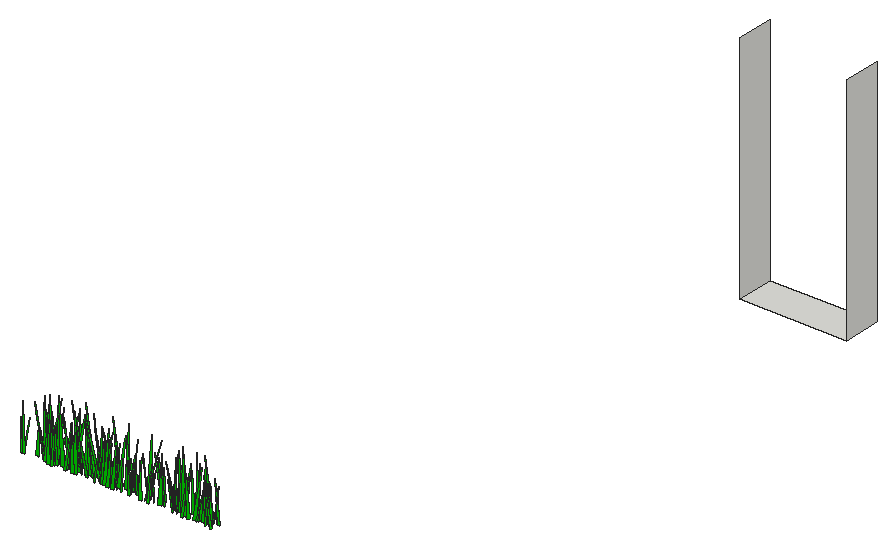
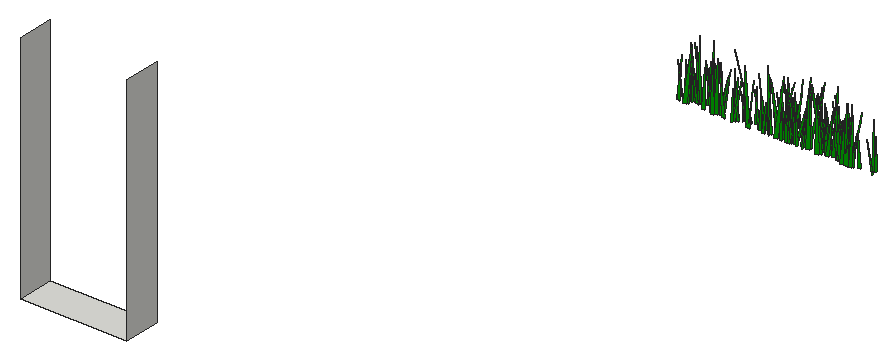
# SketchUp Ruby script. Lengths in inches.
U = 1.inch
M = Sketchup.active_model
def pt(a) = Geom::Point3d.new(a.map { |v| v * U })
def face(e, loops, mat)
  f = e.add_face(loops[0].map { |a| pt(a) })
  loops[1..].each { |l| e.add_face(l.map { |a| pt(a) }).erase! }
  f.material = f.back_material = mat if mat
  f
end
# faces: each face lists its corners as indices into pts; further lists are holes
def faces(e, pts, list, mat = nil) = list.each { |f| face(e, (f[0].is_a?(Array) ? f : [f]).map { |l| l.map { |i| pts[i] } }, mat) }
# xy, xz, yz: faces in a plane at the given z, y or x. An outline is a flat list of corners, or four numbers for a rectangle; further outlines are holes
def ring(l) = l.size == 4 ? [[l[0], l[1]], [l[2], l[1]], [l[2], l[3]], [l[0], l[3]]] : l.each_slice(2).to_a
def flat(e, list, mat, &to3) = list.each { |f| face(e, (f[0].is_a?(Array) ? f : [f]).map { |l| ring(l).map { |u, v| to3.(u, v) } }, mat) }
def xy(e, z, list, mat = nil) = flat(e, list, mat) { |x, y| [x, y, z] }
def xz(e, y, list, mat = nil) = flat(e, list, mat) { |x, z| [x, y, z] }
def yz(e, x, list, mat = nil) = flat(e, list, mat) { |y, z| [x, y, z] }
def lines(e, pts, list) = list.each { |a, b| e.add_line(pt(pts[a]), pt(pts[b])) }
# prism: a flat outline (further loops are holes) pulled along v
def prism(e, loops, v, mat = nil)
  f = face(e, loops, mat); d = Geom::Vector3d.new(v.map { |x| x * U })
  f.pushpull(f.normal.samedirection?(d) ? d.length : -d.length)
end
def box(e, o, s, mat = nil) = prism(e, [[o, [o[0] + s[0], o[1], o[2]], [o[0] + s[0], o[1] + s[1], o[2]], [o[0], o[1] + s[1], o[2]]]], [0, 0, s[2]], mat)
def at(x, y, z, deg = 0) = Geom::Transformation.translation(pt([x, y, z])) * Geom::Transformation.rotation(ORIGIN, Z_AXIS, deg.degrees)
def axes(o, x, y, z) = Geom::Transformation.new([*x, 0, *y, 0, *z, 0, *pt(o).to_a, 1])
def part(name) = M.definitions.add(name)
# library, detail: a bought-in or finely detailed component or shape, given as its bounding box
def library(name, o, s) = part(name).tap { |d| box(d.entities, o, s) }
def detail(e, o, s) = box(e.add_group.entities, o, s)
def put(e, d, t, mat = nil) = e.add_instance(d, t).tap { |i| i.material = mat if mat }
def group(e, t, mat = nil) = e.add_group.tap { |g| g.transformation = t; g.material = mat if mat }.entities
root = M.entities
M.materials.add("[Color G06]").color = [0, 204, 0]
c1 = part("fur_instance\#9")
p = [[0.8125,0,1.79],[0.67,-0.02,1.48],[0,-0.11,0],[0,0.11,0]]
faces(c1.entities,p,[[0,1,2,3]])
xy(root,4.64,[[144.35,175.125,174.23,185.625]])
yz(root,144.35,[[175.125,4.64,185.625,70.2]])
yz(root,174.23,[[175.125,4.64,185.625,70.2]])
put(root,c1,axes([117.61,23,4.28],[-2.5599,0.32054,0.39993],[2.31118,0.35695,0.17964],[0.11843,-0.03742,5.13894]),"[Color G06]")
put(root,c1,axes([72.84,23.15,4.28],[2.39176,-0.2676,1.34014],[-1.98531,-0.34895,-0.08977],[-0.73841,0.07143,4.58218]),"[Color G06]")
put(root,c1,axes([84.67,23.125,4.28],[2.95899,0.07959,1.00137],[0.60026,-0.42215,-0.10781],[-0.64369,-0.02781,4.50266]),"[Color G06]")
put(root,c1,axes([99.72,23.21,4.28],[2.01452,-0.26444,1.03727],[-1.95316,-0.28988,-0.01622],[-0.51301,0.0652,4.135]),"[Color G06]")
put(root,c1,axes([115.85,23.19,4.28],[-2.65021,0.2148,1.87506],[1.74432,0.39119,0.35918],[0.95084,-0.11895,4.56729]),"[Color G06]")
put(root,c1,axes([88.24,23.3125,4.28],[2.48366,-0.43512,0.95898],[-3.15902,-0.35104,-0.02176],[-0.41112,0.06872,5.96054]),"[Color G06]")
put(root,c1,axes([76.27,23.26,4.28],[2.97995,-0.33517,0.86688],[-2.45565,-0.41597,0.38077],[-0.28869,0.07863,5.70926]),"[Color G06]")
put(root,c1,axes([109.36,23.07,4.28],[0.6028,0.39995,0.34159],[2.87417,-0.0822,-0.27409],[0.1331,-0.0364,4.37174]),"[Color G06]")
put(root,c1,axes([71.66,23.17,4.28],[-1.43471,0.42994,1.50699],[3.19984,0.21282,-0.17016],[0.53282,-0.12042,5.07971]),"[Color G06]")
put(root,c1,axes([89.84,23.08,4.28],[1.51874,0.50728,0.66766],[3.65066,-0.21537,0.24767],[-0.32585,-0.04847,5.88662]),"[Color G06]")
put(root,c1,axes([110.98,23.25,4.28],[-2.84036,0.2913,2.00087],[2.29731,0.41596,0.32806],[0.93728,-0.13677,5.25939]),"[Color G06]")
put(root,c1,axes([87.25,23.33,4.28],[-2.79469,0.4392,4.2365],[3.72814,0.47991,-0.22183],[2.01398,-0.27892,6.2894]),"[Color G06]")
put(root,c1,axes([78.32,23.36,4.28],[0.29829,-0.52756,2.06636],[-4.02276,-0.04888,-0.13656],[-0.20558,0.19108,5.67031]),"[Color G06]")
put(root,c1,axes([89.44,23.41,4.28],[-2.8058,-0.48055,1.79717],[-3.58951,0.40162,-0.1816],[0.66131,0.14106,6.6393]),"[Color G06]")
put(root,c1,axes([94.18,23.34,4.28],[-2.1101,-0.2329,1.69497],[-1.84814,0.3149,-0.16881],[0.81239,0.11146,4.01849]),"[Color G06]")
put(root,c1,axes([106.39,23.42,4.28],[-2.33762,-0.19114,0.64303],[-1.40579,0.32795,-0.21743],[0.2961,0.04802,4.04423]),"[Color G06]")
put(root,c1,axes([97.49,23.3125,4.28],[-0.5252,0.45283,1.11862],[3.33154,0.07389,0.05775],[0.08037,-0.1039,4.91617]),"[Color G06]")
put(root,c1,axes([112.3,23.65,4.28],[3.10487,-0.60042,0.08751],[-4.30615,-0.43296,0.02328],[-0.02161,0.00789,7.93391]),"[Color G06]")
put(root,c1,axes([79.09,23.48,4.28],[2.73116,-0.57067,2.98564],[-4.37171,-0.41953,-0.2786],[-1.27545,0.21596,7.34815]),"[Color G06]")
put(root,c1,axes([73.05,23.31,4.28],[-1.69569,0.40002,0.32371],[2.8636,0.23806,-0.28629],[0.27528,-0.01234,4.97218]),"[Color G06]")
put(root,c1,axes([88.36,23.54,4.28],[2.56578,0.37607,3.21461],[3.01226,-0.42641,0.35992],[-1.68094,-0.19011,5.55175]),"[Color G06]")
put(root,c1,axes([91.88,23.63,4.28],[2.03788,-0.29646,0.84145],[-2.12734,-0.29287,-0.34437],[-0.55775,0.03387,4.38793]),"[Color G06]")
put(root,c1,axes([63.83,23.51,4.28],[2.2039,-0.21291,2.10143],[-1.78737,-0.34006,0.22942],[-1.05518,0.13134,4.00054]),"[Color G06]")
put(root,c1,axes([86.43,23.5,4.28],[-2.44167,-0.2565,2.83012],[-2.24312,0.39123,-0.24954],[1.39201,0.18052,4.56211]),"[Color G06]")
put(root,c1,axes([82.1,23.6875,4.28],[-4.64314,-0.43907,0.64752],[-3.16885,0.64777,-0.29859],[0.24588,0.05701,8.37937]),"[Color G06]")
put(root,c1,axes([107.46,23.6,4.28],[-3.35251,-0.15897,0.34434],[-1.15268,0.4672,-0.29086],[0.15501,0.03608,5.28434]),"[Color G06]")
put(root,c1,axes([109.38,23.45,4.28],[-2.29398,0.72773,2.34567],[5.38397,0.33938,-0.33396],[0.84324,-0.18719,8.51349]),"[Color G06]")
put(root,c1,axes([78.55,23.77,4.28],[4.51424,-0.47738,0.28232],[-3.42474,-0.6299,-0.03153],[-0.16326,0.01357,8.46749]),"[Color G06]")
put(root,c1,axes([90.55,23.625,4.28],[-5.29936,0.01222,0.2267],[0.08741,0.73927,-0.01237],[0.1518,0.0008,7.92136]),"[Color G06]")
put(root,c1,axes([98.36,23.65,4.28],[6.18917,0.0656,0.13916],[0.47387,-0.86239,-0.37808],[-0.07359,-0.03616,9.26914]),"[Color G06]")
put(root,c1,axes([113.07,23.53,4.28],[2.59838,0.28438,0.02851],[2.03238,-0.36141,0.37525],[-0.16998,0.0259,4.92249]),"[Color G06]")
put(root,c1,axes([115.7,23.68,4.28],[2.75461,0.17443,2.20644],[1.41082,-0.42616,-0.06434],[-1.32427,-0.09119,4.5211]),"[Color G06]")
put(root,c1,axes([64.5,23.63,4.28],[-2.96816,0.41781,2.14015],[3.10848,0.44379,-0.32288],[1.16852,-0.11928,6.29513]),"[Color G06]")
put(root,c1,axes([87.4375,23.69,4.28],[-2.98027,0.20442,1.90008],[1.56465,0.44533,-0.02175],[1.14765,-0.0763,4.96387]),"[Color G06]")
put(root,c1,axes([70.33,23.72,4.28],[-4.0538,0.18348,3.82784],[1.40302,0.66444,-0.33958],[2.51442,-0.07494,6.36079]),"[Color G06]")
put(root,c1,axes([116.875,23.62,4.28],[-0.12835,0.48306,0.56522],[3.48458,0.01828,-0.02747],[0.03248,-0.0526,5.18091]),"[Color G06]")
put(root,c1,axes([86.54,23.82,4.28],[4.87915,-0.01885,0.99327],[-0.12733,-0.68662,-0.09972],[-0.66613,-0.00682,7.29437]),"[Color G06]")
put(root,c1,axes([113,23.84,4.28],[3.5428,0.53992,3.61843],[4.24445,-0.54697,0.09275],[-1.68464,-0.24262,7.84323]),"[Color G06]")
put(root,c1,axes([85.75,23.88,4.28],[3.4918,0.04867,1.61056],[0.43542,-0.50724,-0.34774],[-1.04569,-0.04869,5.23322]),"[Color G06]")
put(root,c1,axes([73.4375,23.89,4.28],[-2.37338,0.25729,1.7778],[2.01847,0.35181,0.17021],[0.86325,-0.11522,4.48981]),"[Color G06]")
put(root,c1,axes([93.93,23.86,4.28],[2.75429,-0.38398,3.83172],[-3.35008,-0.45195,0.17627],[-1.7124,0.26657,5.81822]),"[Color G06]")
put(root,c1,axes([80.56,23.96,4.28],[-6.04895,-0.02529,1.8238],[-0.20795,0.86023,-0.17053],[1.21603,0.02132,9.04305]),"[Color G06]")
put(root,c1,axes([69.71,24.09,4.28],[-1.78004,-0.30337,0.47503],[-2.17273,0.25145,0.26042],[0.3366,0.01875,4.19313]),"[Color G06]")
put(root,c1,axes([89.21,24.04,4.28],[2.18577,-0.21646,0.93995],[-1.58102,-0.31425,-0.10069],[-0.55267,0.0429,4.00551]),"[Color G06]")
put(root,c1,axes([74.93,24.22,4.28],[-1.3467,-0.84024,1.52468],[-6.10648,0.19083,0.03274],[0.24417,0.13815,9.22785]),"[Color G06]")
put(root,c1,axes([88.76,24.09,4.28],[-2.07942,-0.3279,1.15131],[-2.37477,0.30387,0.36085],[0.69502,0.05726,4.67753]),"[Color G06]")
put(root,c1,axes([69.97,24.05,4.28],[-4.84878,-0.02816,0.938],[-0.17519,0.68124,0.32664],[0.6356,-0.02706,7.24578]),"[Color G06]")
put(root,c1,axes([98.89,24.06,4.28],[-3.72793,-0.04329,1.4862],[-0.30147,0.53802,0.11098],[0.99715,0.00083,5.58985]),"[Color G06]")
put(root,c1,axes([76.14,23.92,4.28],[1.36909,0.58691,0.09506],[4.20916,-0.19079,-0.09339],[0.03975,-0.01113,6.61423]),"[Color G06]")
put(root,c1,axes([106.54,24.34,4.28],[-3.38436,-0.37645,0.00598],[-2.69604,0.47135,0.32596],[0.13913,-0.02343,6.46208]),"[Color G06]")
put(root,c1,axes([114.72,23.98,4.28],[1.17303,0.70372,1.07038],[5.08413,-0.16884,0.30605],[-0.36337,-0.09067,7.73744]),"[Color G06]")
put(root,c1,axes([106.84,24.3125,4.28],[-1.53866,-0.44725,0.95187],[-3.2292,0.22327,0.39138],[0.51459,0.06381,5.30223]),"[Color G06]")
put(root,c1,axes([88.91,24.2,4.28],[1.79576,0.2418,1.9153],[1.90952,-0.28635,0.15374],[-1.0014,-0.11243,3.72775]),"[Color G06]")
put(root,c1,axes([114.63,24.17,4.28],[-3.18706,0.1035,2.27879],[0.71296,0.49247,-0.34214],[1.53862,-0.01381,4.87879]),"[Color G06]")
put(root,c1,axes([115.71,24.375,4.28],[-0.3016,-0.4986,0.55212],[-3.5893,0.04458,0.2449],[0.19516,0.04935,5.35734]),"[Color G06]")
put(root,c1,axes([100.37,24.26,4.28],[-2.96972,-0.03428,1.75489],[-0.24888,0.44524,0.05842],[1.17354,0.00767,4.45326]),"[Color G06]")
put(root,c1,axes([113,24.23,4.28],[-4.05303,-0.20678,3.44647],[-1.75316,0.63671,-0.21697],[2.10782,0.13198,6.44659]),"[Color G06]")
put(root,c1,axes([85.75,24.32,4.28],[-5.18997,-0.27488,1.84227],[-2.02957,0.74076,-0.07525],[1.13396,0.06775,8.29709]),"[Color G06]")
put(root,c1,axes([73.56,24.25,4.28],[2.69049,0.15872,0.20713],[1.14622,-0.37362,-0.36884],[-0.03091,-0.03923,4.35057]),"[Color G06]")
put(root,c1,axes([88.79,24.27,4.28],[2.55794,0.15734,0.56626],[1.14414,-0.35956,-0.06774],[-0.32814,-0.02716,4.17792]),"[Color G06]")
put(root,c1,axes([107.73,24.39,4.28],[-1.14535,0.46018,3.07666],[3.79808,0.19682,-0.22355],[0.83835,-0.263,5.21605]),"[Color G06]")
put(root,c1,axes([103.24,24.4,4.28],[-2.75886,-0.25135,1.55607],[-1.87261,0.40495,0.09779],[0.90897,0.07138,4.92436]),"[Color G06]")
put(root,c1,axes([81.54,24.3,4.28],[0.50592,0.61722,2.12596],[4.63739,-0.08122,0.24376],[-0.33152,-0.19423,6.65401]),"[Color G06]")
put(root,c1,axes([113.46,24.27,4.28],[0.96738,0.38767,0.31174],[2.78709,-0.13373,-0.21498],[0.06773,-0.03405,4.39416]),"[Color G06]")
put(root,c1,axes([85.29,24.35,4.28],[-5.38822,0.22331,0.07516],[1.6022,0.75082,0.30536],[-0.01004,-0.02931,8.39569]),"[Color G06]")
put(root,c1,axes([102.27,24.19,4.28],[0.65066,0.65996,0.03595],[4.72906,-0.09079,0.27878],[-0.18807,0.00022,7.13452]),"[Color G06]")
put(root,c1,axes([67.5,24.6,4.28],[0.22864,-0.39622,0.60995],[-2.8647,-0.02784,0.32113],[0.18371,0.05899,4.24833]),"[Color G06]")
put(root,c1,axes([90.35,24.34,4.28],[2.83915,0.54653,0.84565],[3.95512,-0.39615,-0.25015],[-0.19527,-0.07764,7.22881]),"[Color G06]")
put(root,c1,axes([77.11,24.45,4.28],[2.98341,-0.21861,2.81273],[-1.91767,-0.46576,0.38502],[-1.52383,0.15814,5.02233]),"[Color G06]")
put(root,c1,axes([85.95,24.67,4.28],[-3.18494,-0.45944,0.4711],[-3.29927,0.44556,0.09351],[0.26415,0.02552,6.84827]),"[Color G06]")
put(root,c1,axes([107.7,24.47,4.28],[3.31788,0.20952,0.06508],[1.5022,-0.4627,0.04798],[-0.05291,0.00157,5.44337]),"[Color G06]")
put(root,c1,axes([76.42,24.51,4.28],[4.9796,0.17635,1.10664],[1.27508,-0.70164,0.0279],[-0.7223,-0.02287,7.67858]),"[Color G06]")
put(root,c1,axes([70.89,24.46,4.28],[0.57605,0.4763,0.65461],[3.43102,-0.08469,0.33416],[-0.29491,-0.05487,5.16632]),"[Color G06]")
put(root,c1,axes([79.05,24.65,4.28],[-1.49114,-0.34433,1.32385],[-2.59194,0.21529,-0.08889],[0.40453,0.1102,4.31027]),"[Color G06]")
put(root,c1,axes([116,24.65,4.28],[-3.5417,-0.23177,1.27947],[-1.73909,0.50227,-0.30124],[0.6863,0.07669,5.83947]),"[Color G06]")
put(root,c1,axes([83.03,24.58,4.28],[-2.47971,0.20071,0.92667],[1.46025,0.35466,-0.09582],[0.56903,-0.03548,4.28413]),"[Color G06]")
put(root,c1,axes([90.32,24.67,4.28],[-2.60091,-0.24776,1.90599],[-1.94655,0.38821,-0.13627],[0.99709,0.11159,4.70573]),"[Color G06]")
put(root,c1,axes([94.09,24.65,4.28],[4.61964,0.04994,1.88172],[0.32091,-0.66756,0.27547],[-1.26904,0.01299,6.91963]),"[Color G06]")
put(root,c1,axes([95.65,24.66,4.28],[2.41199,0.30614,1.1997],[2.26998,-0.34515,-0.07665],[-0.558,-0.08078,4.87398]),"[Color G06]")
put(root,c1,axes([83.55,24.76,4.28],[-5.98442,0.19047,2.0085],[1.44632,0.8521,0.34354],[1.25689,-0.07366,9.16773]),"[Color G06]")
put(root,c1,axes([99.21,24.78,4.28],[2.7154,0.04043,0.60274],[0.29582,-0.38271,-0.02778],[-0.399,-0.00858,4.08134]),"[Color G06]")
put(root,c1,axes([79.73,24.8,4.28],[-3.0244,0.07305,0.11029],[0.52822,0.42023,0.384],[0.0286,-0.03706,4.57139]),"[Color G06]")
put(root,c1,axes([106.09,24.83,4.28],[2.41017,-0.46009,2.45395],[-3.53744,-0.36554,-0.11224],[-1.0337,0.17819,6.10574]),"[Color G06]")
put(root,c1,axes([95.31,24.81,4.28],[1.61229,-0.25452,1.94053],[-2.01281,-0.26251,-0.21964],[-0.98282,0.12007,3.63321]),"[Color G06]")
put(root,c1,axes([88.8,24.7,4.28],[2.21731,0.4462,0.75612],[3.23855,-0.30745,-0.372],[-0.08125,-0.0778,5.80645]),"[Color G06]")
put(root,c1,axes([92.3,24.89,4.28],[2.86346,-0.65702,2.69477],[-4.96502,-0.41825,0.07073],[-0.89383,0.21846,8.24005]),"[Color G06]")
put(root,c1,axes([85.125,24.93,4.28],[-0.01838,-0.5965,1.69919],[-4.42104,0.01009,0.29999],[0.21256,0.15824,6.38626]),"[Color G06]")
put(root,c1,axes([69.36,25,4.28],[1.35839,-0.39591,0.00678],[-2.83913,-0.18941,0.03446],[0.01884,0.00196,4.70392]),"[Color G06]")
put(root,c1,axes([108.24,24.9,4.28],[4.04824,-0.11308,1.15367],[-0.85326,-0.57307,0.2353],[-0.72486,0.04303,6.1661]),"[Color G06]")
put(root,c1,axes([76.33,24.75,4.28],[-2.71708,0.45907,0.5274],[3.29649,0.38103,-0.16376],[0.30934,-0.02818,6.37756]),"[Color G06]")
put(root,c1,axes([101.33,24.875,4.28],[1.9813,0.31172,1.12863],[2.31245,-0.28386,-0.06167],[-0.46899,-0.08273,4.46399]),"[Color G06]")
put(root,c1,axes([116.125,24.9375,4.28],[-2.10143,-0.26608,1.42529],[-2.06902,0.29967,-0.38757],[0.51916,0.11726,4.22457]),"[Color G06]")
put(root,c1,axes([81.7,24.89,4.28],[-2.08585,0.61709,2.60961],[4.70231,0.30776,0.0356],[0.72156,-0.22174,7.31179]),"[Color G06]")
put(root,c1,axes([73.58,24.9375,4.28],[-3.46109,-0.34535,3.67224],[-2.75104,0.56698,0.33347],[2.14535,0.16989,6.35203]),"[Color G06]")
put(root,c1,axes([116.71,25.03,4.28],[3.29551,0.01778,1.16478],[0.1769,-0.47112,-0.29199],[-0.76963,-0.03217,4.92041]),"[Color G06]")
put(root,c1,axes([69.01,25.05,4.28],[3.80457,-0.43535,2.95482],[-3.36226,-0.57199,-0.01087],[-1.5333,0.17404,7.35564]),"[Color G06]")
put(root,c1,axes([77.9,25.01,4.28],[2.02111,0.41018,1.55017],[3.08411,-0.28854,-0.21135],[-0.46553,-0.13074,5.32989]),"[Color G06]")
put(root,c1,axes([73.3125,24.84,4.28],[-0.32349,0.6979,0.74631],[5.02832,0.04323,0.22416],[-0.11822,-0.07081,7.49239]),"[Color G06]")
put(root,c1,axes([70.23,24.93,4.28],[4.97967,0.45002,0.50107],[3.23913,-0.69448,-0.25474],[-0.18838,-0.04539,8.86512]),"[Color G06]")
put(root,c1,axes([102.13,25.21,4.28],[-1.23419,-0.50822,1.0503],[-3.70918,0.17268,-0.13725],[0.13692,0.09697,5.74929]),"[Color G06]")
put(root,c1,axes([70.26,25.15,4.28],[-3.83056,-0.12046,1.95691],[-0.82278,0.56449,0.39423],[1.33555,0.00225,5.85558]),"[Color G06]")
put(root,c1,axes([79.19,25.2,4.28],[1.33974,-0.32065,0.83905],[-2.32278,-0.19541,-0.29391],[-0.4555,0.05335,3.96664]),"[Color G06]")
put(root,c1,axes([63.48,25.17,4.28],[2.73976,-0.10168,0.84116],[-0.77809,-0.38728,0.28305],[-0.493,0.04616,4.22785]),"[Color G06]")
put(root,c1,axes([84.48,25.26,4.28],[1.86667,-0.26884,1.04234],[-1.94753,-0.27361,-0.31604],[-0.64058,0.04846,3.99825]),"[Color G06]")
put(root,c1,axes([115.01,25.3,4.28],[1.90158,-0.36385,1.14794],[-2.64708,-0.27761,-0.31335],[-0.62558,0.06868,4.81533]),"[Color G06]")
put(root,c1,axes([117.9,25.26,4.28],[-2.9081,-0.32683,1.65738],[-2.4639,0.42071,-0.12669],[0.80771,0.10661,5.58086]),"[Color G06]")
put(root,c1,axes([85.88,25.27,4.28],[-2.97234,0.07216,1.43601],[0.47212,0.4355,-0.33106],[0.98389,0.00902,4.49704]),"[Color G06]")
put(root,c1,axes([108.77,25.3,4.28],[3.95562,0.17732,1.77731],[1.31721,-0.57398,0.02972],[-1.13843,-0.048,6.20986]),"[Color G06]")
put(root,c1,axes([117.57,25.43,4.28],[0.88785,-0.38657,1.31623],[-2.86527,-0.13834,-0.35025],[-0.50091,0.10616,4.33644]),"[Color G06]")
put(root,c1,axes([71.42,25.3,4.28],[1.04079,0.44341,0.75927],[3.21905,-0.14135,-0.37414],[0.08305,-0.07812,4.98652]),"[Color G06]")
put(root,c1,axes([102.29,25.31,4.28],[-3.5332,0.32381,0.34415],[2.32388,0.49355,-0.05176],[0.21147,-0.01359,6.31878]),"[Color G06]")
put(root,c1,axes([93.71,25.34,4.28],[-0.24196,0.4314,0.8795],[3.13327,0.04123,-0.39764],[0.31569,-0.07856,4.62074]),"[Color G06]")
put(root,c1,axes([110.65,25.32,4.28],[-1.49834,0.48574,0.86116],[3.50624,0.21497,-0.30173],[0.41493,-0.06245,5.65932]),"[Color G06]")
put(root,c1,axes([93.91,25.44,4.28],[-2.33062,0.17922,0.94591],[1.31202,0.3347,-0.06375],[0.57531,-0.03726,3.9773]),"[Color G06]")
put(root,c1,axes([69.4,25.46,4.28],[-3.19656,0.40574,2.04489],[3.07719,0.46406,0.16749],[0.93234,-0.14051,6.45818]),"[Color G06]")
put(root,c1,axes([70.6,25.59,4.28],[1.17832,0.64638,3.72469],[5.20592,-0.19538,0.21616],[-0.77176,-0.33105,7.14493]),"[Color G06]")
put(root,c1,axes([88.8,25.5625,4.28],[3.31252,0.28199,2.58576],[2.2308,-0.50427,-0.06618],[-1.45131,-0.13147,5.80009]),"[Color G06]")
put(root,c1,axes([70.6,25.47,4.28],[-1.98355,0.4542,0.97916],[3.29975,0.28172,-0.08019],[0.38722,-0.07407,5.69914]),"[Color G06]")
put(root,c1,axes([71.7,25.48,4.28],[-1.63826,0.51749,1.11996],[3.77855,0.23062,0.10505],[0.23719,-0.0996,6.06199]),"[Color G06]")
put(root,c1,axes([90.29,25.46,4.28],[-3.93521,0.58747,1.25479],[4.27647,0.55077,0.33672],[0.40628,-0.10716,8.60951]),"[Color G06]")
put(root,c1,axes([108.02,25.51,4.28],[-0.1711,0.63969,1.9554],[4.77025,0.02181,0.11293],[-0.02975,-0.1827,6.86008]),"[Color G06]")
put(root,c1,axes([108.07,25.59,4.28],[1.24459,0.35005,1.42046],[2.67833,-0.17162,-0.38362],[-0.17756,-0.13503,4.17005]),"[Color G06]")
put(root,c1,axes([104.93,25.59,4.28],[-2.57655,-0.39735,3.8404],[-3.3899,0.43792,0.12469],[1.79743,0.25632,5.74024]),"[Color G06]")
put(root,c1,axes([87.27,25.67,4.28],[-1.58635,-0.41634,2.28109],[-3.26468,0.2455,0.07573],[0.76514,0.18429,5.05248]),"[Color G06]")
put(root,c1,axes([107.13,25.51,4.28],[-1.64359,0.65776,1.26388],[4.78379,0.23258,-0.00854],[0.28372,-0.11109,7.4656]),"[Color G06]")
put(root,c1,axes([92.12,25.7,4.28],[-2.95123,-0.00697,1.76936],[-0.00421,0.44313,0.18479],[1.1849,-0.01578,4.40759]),"[Color G06]")
put(root,c1,axes([82.71,25.7,4.28],[-3.60138,0.0738,1.4752],[0.59002,0.51898,0.23489],[0.95196,-0.04246,5.43527]),"[Color G06]")
put(root,c1,axes([86.5,25.65,4.28],[1.96222,0.26527,0.94074],[1.94421,-0.28178,0.0692],[-0.48493,-0.05633,4.08407]),"[Color G06]")
put(root,c1,axes([78.77,25.52,4.28],[-1.06123,0.73347,0.78161],[5.27977,0.15065,-0.22682],[0.25286,-0.06725,8.01649]),"[Color G06]")
put(root,c1,axes([107.78,25.74,4.28],[1.3939,0.46367,1.83934],[3.49355,-0.21107,0.19831],[-0.60477,-0.1506,5.38491]),"[Color G06]")
put(root,c1,axes([102.33,25.73,4.28],[-1.05605,0.38226,0.80624],[2.7821,0.15126,-0.09866],[0.2565,-0.06681,4.3895]),"[Color G06]")
put(root,c1,axes([115.6875,25.69,4.28],[-3.78492,0.55398,1.12686],[4.01347,0.53222,0.05546],[0.49294,-0.07972,8.20067]),"[Color G06]")
put(root,c1,axes([97.9,25.69,4.28],[1.84702,0.71701,1.27616],[5.19175,-0.26428,0.27287],[-0.46241,-0.10328,8.16113]),"[Color G06]")
